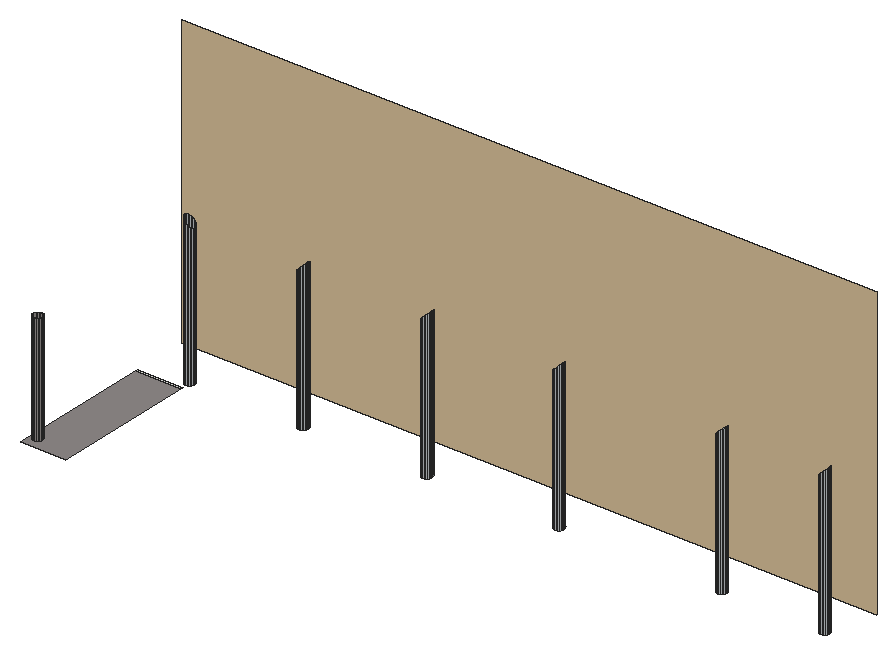
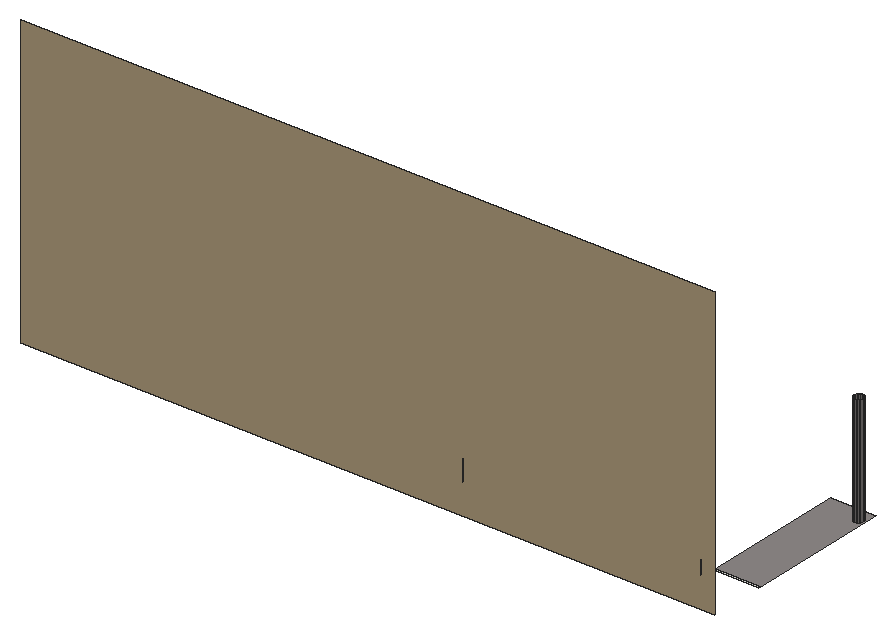
# SketchUp Ruby script. Lengths in inches.
U = 1.inch
M = Sketchup.active_model
def pt(a) = Geom::Point3d.new(a.map { |v| v * U })
def face(e, loops, mat)
  f = e.add_face(loops[0].map { |a| pt(a) })
  loops[1..].each { |l| e.add_face(l.map { |a| pt(a) }).erase! }
  f.material = f.back_material = mat if mat
  f
end
# faces: each face lists its corners as indices into pts; further lists are holes
def faces(e, pts, list, mat = nil) = list.each { |f| face(e, (f[0].is_a?(Array) ? f : [f]).map { |l| l.map { |i| pts[i] } }, mat) }
# xy, xz, yz: faces in a plane at the given z, y or x. An outline is a flat list of corners, or four numbers for a rectangle; further outlines are holes
def ring(l) = l.size == 4 ? [[l[0], l[1]], [l[2], l[1]], [l[2], l[3]], [l[0], l[3]]] : l.each_slice(2).to_a
def flat(e, list, mat, &to3) = list.each { |f| face(e, (f[0].is_a?(Array) ? f : [f]).map { |l| ring(l).map { |u, v| to3.(u, v) } }, mat) }
def xy(e, z, list, mat = nil) = flat(e, list, mat) { |x, y| [x, y, z] }
def xz(e, y, list, mat = nil) = flat(e, list, mat) { |x, z| [x, y, z] }
def yz(e, x, list, mat = nil) = flat(e, list, mat) { |y, z| [x, y, z] }
def lines(e, pts, list) = list.each { |a, b| e.add_line(pt(pts[a]), pt(pts[b])) }
# prism: a flat outline (further loops are holes) pulled along v
def prism(e, loops, v, mat = nil)
  f = face(e, loops, mat); d = Geom::Vector3d.new(v.map { |x| x * U })
  f.pushpull(f.normal.samedirection?(d) ? d.length : -d.length)
end
def box(e, o, s, mat = nil) = prism(e, [[o, [o[0] + s[0], o[1], o[2]], [o[0] + s[0], o[1] + s[1], o[2]], [o[0], o[1] + s[1], o[2]]]], [0, 0, s[2]], mat)
def at(x, y, z, deg = 0) = Geom::Transformation.translation(pt([x, y, z])) * Geom::Transformation.rotation(ORIGIN, Z_AXIS, deg.degrees)
def axes(o, x, y, z) = Geom::Transformation.new([*x, 0, *y, 0, *z, 0, *pt(o).to_a, 1])
def part(name) = M.definitions.add(name)
# library, detail: a bought-in or finely detailed component or shape, given as its bounding box
def library(name, o, s) = part(name).tap { |d| box(d.entities, o, s) }
def detail(e, o, s) = box(e.add_group.entities, o, s)
def put(e, d, t, mat = nil) = e.add_instance(d, t).tap { |i| i.material = mat if mat }
def group(e, t, mat = nil) = e.add_group.tap { |g| g.transformation = t; g.material = mat if mat }.entities
root = M.entities
M.materials.add("[0032_Moccasin]").color = [214, 191, 152]
M.materials.add("[Steel Brushed Stainless]").color = [183, 187, 190]
M.materials.add("[Stone Marble]").color = [143, 138, 136]
xy(root,168,[[672,97.2,690.7,98.16],[690.43,100.13,689.91,100.2,689.42,100.39,689.01,100.7,688.68,101.12,688.48,101.6,688.4,102.11,688.47,102.63,688.66,103.12,688.97,103.53,689.38,103.86,689.86,104.0625,690.38,104.13,690.9,104.07,691.38,103.88,691.8,103.56,692.125,103.15,692.33,102.67,692.4,102.16,692.34,101.64,692.15,101.15,691.83,100.74,691.42,100.41,690.94,100.21],[954.05,100.13,954.29,100.17,954.03,100.14],[953.77,100.17,953.51,100.21,953.53,100.2],[954.55,100.21,954.57,100.21,954.79,100.3],
  [953.27,100.3,953.03,100.41,953.05,100.39],[955.03,100.41,955.05,100.41,955.24,100.5625],[952.82,100.5625,952.62,100.72,952.63,100.7],[955.44,100.72,955.46,100.74,955.6,100.93],[952.46,100.93,952.3,101.14,952.31,101.12],
  [955.76,101.14,955.77,101.15,955.86,101.375],[952.2,101.375,952.1,101.62,952.1,101.6],[955.96,101.62,955.97,101.64,955.99,101.875],[952.0625,101.875,952.03,102.13,952.03,102.11],[956.03,102.13,956.03,102.16,955.99,102.39],
  [952.0625,102.39,952.1,102.65,952.09,102.63],[955.96,102.65,955.95,102.67,955.86,102.89],[952.2,102.89,952.3,103.13,952.29,103.12],[955.76,103.13,955.75,103.15,955.6,103.34],[952.46,103.34,952.62,103.55,952.6,103.53],
  [955.44,103.55,955.43,103.56,955.24,103.71],[952.82,103.71,953.03,103.86,953.01,103.86],[955.03,103.86,955.01,103.88,954.79,103.97],[953.27,103.97,953.51,104.0625,953.49,104.0625],[954.55,104.0625,954.52,104.07,954.29,104.1],
  [953.77,104.1,954.03,104.13,954.01,104.13]])
xy(root,168,[[[672,37.2,690.7,97.2],[674.75,40.78,674.23,40.84,673.75,41.04,673.33,41.36,673.01,41.78,672.8125,42.26,672.75,42.78,672.8125,43.29,673.01,43.78,673.33,44.19,673.75,44.51,674.23,44.71,674.75,44.78,675.26,44.71,675.75,44.51,676.16,44.19,676.48,43.78,676.68,43.29,676.75,42.78,676.68,42.26,676.48,41.78,676.16,41.36,675.75,41.04,675.26,40.84]],[674.75,40.78,674.23,40.84,673.75,41.04,673.33,41.36,673.01,41.78,672.8125,42.26,672.75,42.78,672.8125,43.29,673.01,43.78,673.33,44.19,673.75,44.51,674.23,44.71,674.75,44.78,675.26,44.71,675.75,44.51,676.16,44.19,676.48,43.78,676.68,43.29,676.75,42.78,676.68,42.26,676.48,41.78,676.16,41.36,675.75,41.04,675.26,40.84]],"[Stone Marble]")
xz(root,121.2,[[672,168,960,288]],"[0032_Moccasin]")
p = [[673.75,41.04,168],[674.23,40.84,168],[674.23,40.84,213.56],[673.75,41.04,213.56],[674.75,40.78,168],[674.75,40.78,213.56],
  [675.26,40.84,168],[675.26,40.84,213.56],[675.75,41.04,168],[675.75,41.04,213.56],[673.33,41.36,168],[673.33,41.36,213.56],
  [676.16,41.36,168],[676.16,41.36,213.56],[673.01,41.78,168],[673.01,41.78,213.56],[676.48,41.78,168],[676.48,41.78,213.56],
  [672.8125,42.26,168],[672.8125,42.26,213.56],[676.68,42.26,168],[676.68,42.26,213.56],[676.75,42.78,168],[676.75,42.78,213.56],
  [676.68,43.29,168],[676.68,43.29,213.56],[673.01,43.78,168],[672.8125,43.29,168],[672.8125,43.29,213.56],[673.01,43.78,213.56],
  [676.48,43.78,168],[676.48,43.78,213.56],[673.33,44.19,168],[673.33,44.19,213.56],[676.16,44.19,168],[676.16,44.19,213.56],
  [673.75,44.51,168],[673.75,44.51,213.56],[675.75,44.51,168],[675.75,44.51,213.56],[674.23,44.71,168],[674.23,44.71,213.56],
  [675.26,44.71,168],[675.26,44.71,213.56],[674.75,44.78,168],[674.75,44.78,213.56],[689.91,100.2,168],[690.43,100.13,168],
  [690.43,100.13,227.98],[689.91,100.2,228.5],[690.94,100.21,168],[690.94,100.21,227.46],[737.51,100.13,227.98],[736.99,100.21,227.46],
  [736.99,100.21,168],[737.01,100.21,168],[737.27,100.17,168],[737.51,100.13,168],[738.02,100.2,228.5],[737.53,100.14,168],
  [737.79,100.17,168],[738.02,100.2,168],[788.88,100.13,227.98],[788.36,100.21,227.46],[788.36,100.21,168],[788.39,100.21,168],
  [788.64,100.17,168],[788.88,100.13,168],[789.4,100.2,228.5],[788.9,100.14,168],[789.16,100.17,168],[789.4,100.2,168],
  [843.63,100.13,227.98],[843.11,100.21,227.46],[843.11,100.21,168],[843.14,100.21,168],[843.39,100.17,168],[843.63,100.13,168],
  [844.15,100.2,228.5],[843.65,100.14,168],[843.91,100.17,168],[844.15,100.2,168],[911.13,100.13,227.98],[910.61,100.21,227.46],
  [910.61,100.21,168],[910.64,100.21,168],[910.89,100.17,168],[911.13,100.13,168],[911.65,100.2,228.5],[911.15,100.14,168],
  [911.41,100.17,168],[911.65,100.2,168],[954.01,100.13,227.98],[953.49,100.21,227.46],[953.49,100.21,168],[953.51,100.21,168],
  [953.77,100.17,168],[954.01,100.13,168],[954.52,100.2,228.5],[954.03,100.14,168],[954.29,100.17,168],[954.52,100.2,168],
  [689.42,100.39,168],[689.42,100.39,228.98],[691.42,100.41,168],[691.42,100.41,226.98],[736.51,100.41,226.98],[736.51,100.41,168],
  [736.53,100.41,168],[736.77,100.3,168],[738.51,100.39,228.98],[738.05,100.21,168],[738.29,100.3,168],[738.51,100.39,168],
  [787.88,100.41,226.98],[787.88,100.41,168],[787.9,100.41,168],[788.14,100.3,168],[789.88,100.39,228.98],[789.42,100.21,168],
  [789.66,100.3,168],[789.88,100.39,168],[842.63,100.41,226.98],[842.63,100.41,168],[842.65,100.41,168],[842.89,100.3,168],
  [844.63,100.39,228.98],[844.17,100.21,168],[844.41,100.3,168],[844.63,100.39,168],[910.13,100.41,226.98],[910.13,100.41,168],
  [910.15,100.41,168],[910.39,100.3,168],[912.13,100.39,228.98],[911.67,100.21,168],[911.91,100.3,168],[912.13,100.39,168],
  [953.01,100.41,226.98],[953.01,100.41,168],[953.03,100.41,168],[953.27,100.3,168],[955.01,100.39,228.98],[954.55,100.21,168],
  [954.79,100.3,168],[955.01,100.39,168],[689.01,100.7,168],[689.01,100.7,229.4],[691.83,100.74,168],[691.83,100.74,226.57],
  [736.1,100.74,226.57],[736.1,100.74,168],[736.12,100.72,168],[736.32,100.5625,168],[738.93,100.7,229.4],[738.53,100.41,168],
  [738.74,100.5625,168],[738.93,100.7,168],[787.47,100.74,226.57],[787.47,100.74,168],[787.49,100.72,168],[787.7,100.5625,168],
  [790.3,100.7,229.4],[789.9,100.41,168],[790.11,100.5625,168],[790.3,100.7,168],[842.22,100.74,226.57],[842.22,100.74,168],
  [842.24,100.72,168],[842.45,100.5625,168],[845.05,100.7,229.4],[844.65,100.41,168],[844.86,100.5625,168],[845.05,100.7,168],
  [909.72,100.74,226.57],[909.72,100.74,168],[909.74,100.72,168],[909.95,100.5625,168],[912.55,100.7,229.4],[912.15,100.41,168],
  [912.36,100.5625,168],[912.55,100.7,168],[952.6,100.74,226.57],[952.6,100.74,168],[952.62,100.72,168],[952.82,100.5625,168],
  [955.43,100.7,229.4],[955.03,100.41,168],[955.24,100.5625,168],[955.43,100.7,168],[688.68,101.12,168],[688.68,101.12,229.72],
  [692.15,101.15,168],[692.15,101.15,226.26],[735.79,101.15,226.26],[735.79,101.15,168],[735.8,101.14,168],[735.96,100.93,168],
  [739.25,101.12,229.72],[738.94,100.72,168],[739.1,100.93,168],[739.25,101.12,168],[787.16,101.15,226.26],[787.16,101.15,168],
  [787.17,101.14,168],[787.33,100.93,168],[790.625,101.12,229.72],[790.32,100.72,168],[790.48,100.93,168],[790.625,101.12,168],
  [841.91,101.15,226.26],[841.91,101.15,168],[841.92,101.14,168],[842.08,100.93,168],[845.375,101.12,229.72],[845.07,100.72,168],
  [845.23,100.93,168],[845.375,101.12,168],[909.41,101.15,226.26],[909.41,101.15,168],[909.42,101.14,168],[909.58,100.93,168],
  [912.875,101.12,229.72],[912.57,100.72,168],[912.73,100.93,168],[912.875,101.12,168],[952.29,101.15,226.26],[952.29,101.15,168],
  [952.3,101.14,168],[952.46,100.93,168],[955.75,101.12,229.72],[955.44,100.72,168],[955.6,100.93,168],[955.75,101.12,168],
  [688.48,101.6,168],[688.48,101.6,229.93],[739.45,101.6,229.93],[739.26,101.14,168],[739.36,101.375,168],[739.45,101.6,168],
  [790.83,101.6,229.93],[790.63,101.14,168],[790.74,101.375,168],[790.83,101.6,168],[845.58,101.6,229.93],[845.38,101.14,168],
  [845.49,101.375,168],[845.58,101.6,168],[913.08,101.6,229.93],[912.88,101.14,168],[912.99,101.375,168],[913.08,101.6,168],
  [955.95,101.6,229.93],[955.76,101.14,168],[955.86,101.375,168],[955.95,101.6,168],[692.34,101.64,168],[692.34,101.64,226.0625],
  [735.59,101.64,226.0625],[735.59,101.64,168],[735.6,101.62,168],[735.7,101.375,168],[786.97,101.64,226.0625],[786.97,101.64,168],
  [786.97,101.62,168],[787.07,101.375,168],[841.72,101.64,226.0625],[841.72,101.64,168],[841.72,101.62,168],[841.82,101.375,168],
  [909.22,101.64,226.0625],[909.22,101.64,168],[909.22,101.62,168],[909.32,101.375,168],[952.09,101.64,226.0625],[952.09,101.64,168],
  [952.1,101.62,168],[952.2,101.375,168],[688.4,102.11,168],[688.4,102.11,230],[692.4,102.16,168],[692.4,102.16,226],
  [735.53,102.16,226],[735.53,102.16,168],[735.53,102.13,168],[735.5625,101.875,168],[739.53,102.11,230],[739.46,101.62,168],
  [739.49,101.875,168],[739.53,102.11,168],[786.9,102.16,226],[786.9,102.16,168],[786.91,102.13,168],[786.9375,101.875,168],
  [790.9,102.11,230],[790.83,101.62,168],[790.87,101.875,168],[790.9,102.11,168],[841.65,102.16,226],[841.65,102.16,168],
  [841.66,102.13,168],[841.6875,101.875,168],[845.65,102.11,230],[845.58,101.62,168],[845.62,101.875,168],[845.65,102.11,168],
  [909.15,102.16,226],[909.15,102.16,168],[909.16,102.13,168],[909.1875,101.875,168],[913.15,102.11,230],[913.08,101.62,168],
  [913.12,101.875,168],[913.15,102.11,168],[952.03,102.16,226],[952.03,102.16,168],[952.03,102.13,168],[952.0625,101.875,168],
  [956.03,102.11,230],[955.96,101.62,168],[955.99,101.875,168],[956.03,102.11,168],[688.47,102.63,168],[688.47,102.63,229.9375],
  [739.47,102.63,229.9375],[739.53,102.13,168],[739.49,102.39,168],[739.47,102.63,168],[790.84,102.63,229.9375],[790.9,102.13,168],
  [790.87,102.39,168],[790.84,102.63,168],[845.59,102.63,229.9375],[845.65,102.13,168],[845.62,102.39,168],[845.59,102.63,168],
  [913.09,102.63,229.9375],[913.15,102.13,168],[913.12,102.39,168],[913.09,102.63,168],[955.97,102.63,229.9375],[956.03,102.13,168],
  [955.99,102.39,168],[955.97,102.63,168],[692.33,102.67,168],[692.33,102.67,226.07],[735.6,102.67,226.07],[735.6,102.67,168],
  [735.6,102.65,168],[735.5625,102.39,168],[786.98,102.67,226.07],[786.98,102.67,168],[786.97,102.65,168],[786.9375,102.39,168],
  [841.73,102.67,226.07],[841.73,102.67,168],[841.72,102.65,168],[841.6875,102.39,168],[909.23,102.67,226.07],[909.23,102.67,168],
  [909.22,102.65,168],[909.1875,102.39,168],[952.1,102.67,226.07],[952.1,102.67,168],[952.1,102.65,168],[952.0625,102.39,168],
  [688.66,103.12,168],[688.66,103.12,229.74],[739.27,103.12,229.74],[739.46,102.65,168],[739.36,102.89,168],[739.27,103.12,168],
  [790.65,103.12,229.74],[790.83,102.65,168],[790.74,102.89,168],[790.65,103.12,168],[845.4,103.12,229.74],[845.58,102.65,168],
  [845.49,102.89,168],[845.4,103.12,168],[912.9,103.12,229.74],[913.08,102.65,168],[912.99,102.89,168],[912.9,103.12,168],
  [955.77,103.12,229.74],[955.96,102.65,168],[955.86,102.89,168],[955.77,103.12,168],[692.125,103.15,168],[692.125,103.15,226.28],
  [735.81,103.15,226.28],[735.81,103.15,168],[735.8,103.13,168],[735.7,102.89,168],[787.18,103.15,226.28],[787.18,103.15,168],
  [787.17,103.13,168],[787.07,102.89,168],[841.93,103.15,226.28],[841.93,103.15,168],[841.92,103.13,168],[841.82,102.89,168],
  [909.43,103.15,226.28],[909.43,103.15,168],[909.42,103.13,168],[909.32,102.89,168],[952.31,103.15,226.28],[952.31,103.15,168],
  [952.3,103.13,168],[952.2,102.89,168],[688.97,103.53,168],[688.97,103.53,229.43],[738.96,103.53,229.43],[739.26,103.13,168],
  [739.1,103.34,168],[738.96,103.53,168],[790.33,103.53,229.43],[790.63,103.13,168],[790.48,103.34,168],[790.33,103.53,168],
  [845.08,103.53,229.43],[845.38,103.13,168],[845.23,103.34,168],[845.08,103.53,168],[912.58,103.53,229.43],[912.88,103.13,168],
  [912.73,103.34,168],[912.58,103.53,168],[955.46,103.53,229.43],[955.76,103.13,168],[955.6,103.34,168],[955.46,103.53,168],
  [691.8,103.56,168],[691.8,103.56,226.6],[736.13,103.56,226.6],[736.13,103.56,168],[736.12,103.55,168],[735.96,103.34,168],
  [787.51,103.56,226.6],[787.51,103.56,168],[787.49,103.55,168],[787.33,103.34,168],[842.26,103.56,226.6],[842.26,103.56,168],
  [842.24,103.55,168],[842.08,103.34,168],[909.76,103.56,226.6],[909.76,103.56,168],[909.74,103.55,168],[909.58,103.34,168],
  [952.63,103.56,226.6],[952.63,103.56,168],[952.62,103.55,168],[952.46,103.34,168],[689.38,103.86,168],[689.38,103.86,229.02],
  [738.55,103.86,229.02],[738.94,103.55,168],[738.74,103.71,168],[738.55,103.86,168],[789.92,103.86,229.02],[790.32,103.55,168],
  [790.11,103.71,168],[789.92,103.86,168],[844.67,103.86,229.02],[845.07,103.55,168],[844.86,103.71,168],[844.67,103.86,168],
  [912.17,103.86,229.02],[912.57,103.55,168],[912.36,103.71,168],[912.17,103.86,168],[955.05,103.86,229.02],[955.44,103.55,168],
  [955.24,103.71,168],[955.05,103.86,168],[691.38,103.88,168],[691.38,103.88,227.02],[736.55,103.88,227.02],[736.55,103.88,168],
  [736.53,103.86,168],[736.32,103.71,168],[787.92,103.88,227.02],[787.92,103.88,168],[787.9,103.86,168],[787.7,103.71,168],
  [842.67,103.88,227.02],[842.67,103.88,168],[842.65,103.86,168],[842.45,103.71,168],[910.17,103.88,227.02],[910.17,103.88,168],
  [910.15,103.86,168],[909.95,103.71,168],[953.05,103.88,227.02],[953.05,103.88,168],[953.03,103.86,168],[952.82,103.71,168],
  [689.86,104.0625,168],[689.86,104.0625,228.54],[690.9,104.07,168],[690.9,104.07,227.5],[737.03,104.07,227.5],[737.03,104.07,168],
  [737.01,104.0625,168],[736.77,103.97,168],[738.07,104.0625,228.54],[738.53,103.86,168],[738.29,103.97,168],[738.07,104.0625,168],
  [788.41,104.07,227.5],[788.41,104.07,168],[788.39,104.0625,168],[788.14,103.97,168],[789.44,104.0625,228.54],[789.9,103.86,168],
  [789.66,103.97,168],[789.44,104.0625,168],[843.16,104.07,227.5],[843.16,104.07,168],[843.14,104.0625,168],[842.89,103.97,168],
  [844.19,104.0625,228.54],[844.65,103.86,168],[844.41,103.97,168],[844.19,104.0625,168],[910.66,104.07,227.5],[910.66,104.07,168],
  [910.64,104.0625,168],[910.39,103.97,168],[911.69,104.0625,228.54],[912.15,103.86,168],[911.91,103.97,168],[911.69,104.0625,168],
  [953.53,104.07,227.5],[953.53,104.07,168],[953.51,104.0625,168],[953.27,103.97,168],[954.57,104.0625,228.54],[955.03,103.86,168],
  [954.79,103.97,168],[954.57,104.0625,168],[690.38,104.13,168],[690.38,104.13,228.02],[737.55,104.13,228.02],[737.55,104.13,168],
  [737.53,104.13,168],[737.27,104.1,168],[738.05,104.0625,168],[737.79,104.1,168],[788.93,104.13,228.02],[788.93,104.13,168],
  [788.9,104.13,168],[788.64,104.1,168],[789.42,104.0625,168],[789.16,104.1,168],[843.68,104.13,228.02],[843.68,104.13,168],
  [843.65,104.13,168],[843.39,104.1,168],[844.17,104.0625,168],[843.91,104.1,168],[911.18,104.13,228.02],[911.18,104.13,168],
  [911.15,104.13,168],[910.89,104.1,168],[911.67,104.0625,168],[911.41,104.1,168],[954.05,104.13,228.02],[954.05,104.13,168],
  [954.03,104.13,168],[953.77,104.1,168],[954.55,104.0625,168],[954.29,104.1,168],[954.03,102.13,168],[954.03,102.13,228],
  [690.4,102.13,168],[690.4,102.13,228],[674.75,42.78,213.56],[674.75,42.78,168]]
faces(root,p,[[0,1,2,3],[1,4,5,2],[4,6,7,5],[6,8,9,7],[10,0,3,11],[8,12,13,9],[14,10,11,15],[12,16,17,13],
  [18,14,15,19],[16,20,21,17],[20,22,23,21],[22,24,25,23],[26,27,28,29],[24,30,31,25],[32,26,29,33],[30,34,35,31],
  [36,32,33,37],[34,38,39,35],[40,36,37,41],[38,42,43,39],[44,40,41,45],[42,44,45,43]],"[Stone Marble]")
faces(root,p,[[46,47,48,49],[47,50,51,48],[52,53,54,55,56,57],[58,52,57,59,60,61],[62,63,64,65,66,67],[68,62,67,69,70,71],[72,73,74,75,76,77],[78,72,77,79,80,81],
  [82,83,84,85,86,87],[88,82,87,89,90,91],[92,93,94,95,96,97],[98,92,97,99,100,101],[102,46,49,103],[50,104,105,51],[53,106,107,108,109,54],[110,58,61,111,112,113],
  [63,114,115,116,117,64],[118,68,71,119,120,121],[73,122,123,124,125,74],[126,78,81,127,128,129],[83,130,131,132,133,84],[134,88,91,135,136,137],[93,138,139,140,141,94],[142,98,101,143,144,145],
  [146,102,103,147],[104,148,149,105],[106,150,151,152,153,107],[154,110,113,155,156,157],[114,158,159,160,161,115],[162,118,121,163,164,165],[122,166,167,168,169,123],[170,126,129,171,172,173],
  [130,174,175,176,177,131],[178,134,137,179,180,181],[138,182,183,184,185,139],[186,142,145,187,188,189],[190,146,147,191],[148,192,193,149],[150,194,195,196,197,151],[198,154,157,199,200,201],
  [158,202,203,204,205,159],[206,162,165,207,208,209],[166,210,211,212,213,167],[214,170,173,215,216,217],[174,218,219,220,221,175],[222,178,181,223,224,225],[182,226,227,228,229,183],[230,186,189,231,232,233],
  [234,190,191,235],[236,198,201,237,238,239],[240,206,209,241,242,243],[244,214,217,245,246,247],[248,222,225,249,250,251],[252,230,233,253,254,255],[192,256,257,193],[194,258,259,260,261,195],
  [202,262,263,264,265,203],[210,266,267,268,269,211],[218,270,271,272,273,219],[226,274,275,276,277,227],[278,234,235,279],[256,280,281,257],[258,282,283,284,285,259],[286,236,239,287,288,289],
  [262,290,291,292,293,263],[294,240,243,295,296,297],[266,298,299,300,301,267],[302,244,247,303,304,305],[270,306,307,308,309,271],[310,248,251,311,312,313],[274,314,315,316,317,275],[318,252,255,319,320,321],
  [322,278,279,323],[324,286,289,325,326,327],[328,294,297,329,330,331],[332,302,305,333,334,335],[336,310,313,337,338,339],[340,318,321,341,342,343],[280,344,345,281],[282,346,347,348,349,283],
  [290,350,351,352,353,291],[298,354,355,356,357,299],[306,358,359,360,361,307],[314,362,363,364,365,315],[366,322,323,367],[368,324,327,369,370,371],[372,328,331,373,374,375],[376,332,335,377,378,379],
  [380,336,339,381,382,383],[384,340,343,385,386,387],[344,388,389,345],[346,390,391,392,393,347],[350,394,395,396,397,351],[354,398,399,400,401,355],[358,402,403,404,405,359],[362,406,407,408,409,363],
  [410,366,367,411],[412,368,371,413,414,415],[416,372,375,417,418,419],[420,376,379,421,422,423],[424,380,383,425,426,427],[428,384,387,429,430,431],[388,432,433,389],[390,434,435,436,437,391],
  [394,438,439,440,441,395],[398,442,443,444,445,399],[402,446,447,448,449,403],[406,450,451,452,453,407],[454,410,411,455],[456,412,415,457,458,459],[460,416,419,461,462,463],[464,420,423,465,466,467],
  [468,424,427,469,470,471],[472,428,431,473,474,475],[432,476,477,433],[434,478,479,480,481,435],[438,482,483,484,485,439],[442,486,487,488,489,443],[446,490,491,492,493,447],[450,494,495,496,497,451],
  [498,454,455,499],[476,500,501,477],[478,502,503,504,505,479],[506,456,459,507,508,509],[482,510,511,512,513,483],[514,460,463,515,516,517],[486,518,519,520,521,487],[522,464,467,523,524,525],
  [490,526,527,528,529,491],[530,468,471,531,532,533],[494,534,535,536,537,495],[538,472,475,539,540,541],[542,498,499,543],[500,542,543,501],[502,544,545,546,547,503],[544,506,509,548,549,545],
  [510,550,551,552,553,511],[550,514,517,554,555,551],[518,556,557,558,559,519],[556,522,525,560,561,557],[526,562,563,564,565,527],[562,530,533,566,567,563],[534,568,569,570,571,535],[568,538,541,572,573,569]],"[Steel Brushed Stainless]")
lines(root,p,[[574,575],[576,577],[578,579]])
